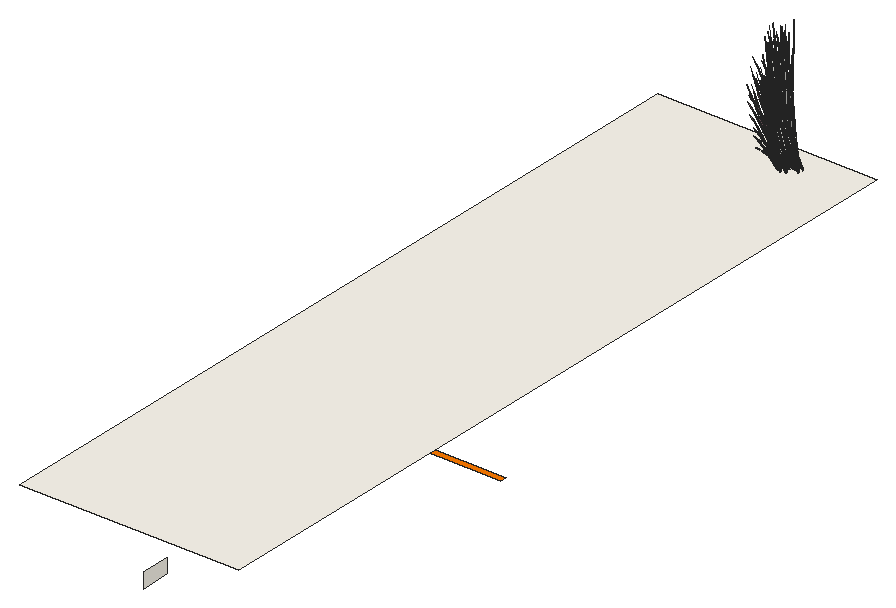
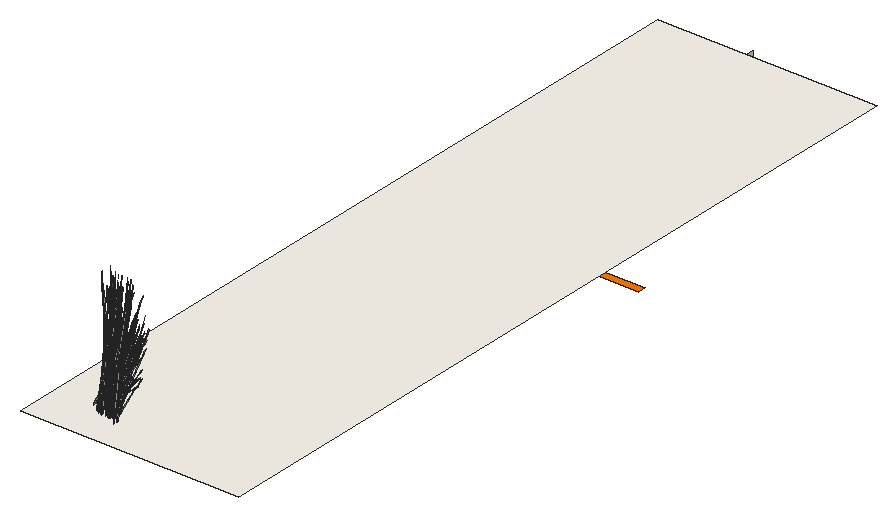
# SketchUp Ruby script. Lengths in inches.
U = 1.inch
M = Sketchup.active_model
def pt(a) = Geom::Point3d.new(a.map { |v| v * U })
def face(e, loops, mat)
  f = e.add_face(loops[0].map { |a| pt(a) })
  loops[1..].each { |l| e.add_face(l.map { |a| pt(a) }).erase! }
  f.material = f.back_material = mat if mat
  f
end
# faces: each face lists its corners as indices into pts; further lists are holes
def faces(e, pts, list, mat = nil) = list.each { |f| face(e, (f[0].is_a?(Array) ? f : [f]).map { |l| l.map { |i| pts[i] } }, mat) }
# xy, xz, yz: faces in a plane at the given z, y or x. An outline is a flat list of corners, or four numbers for a rectangle; further outlines are holes
def ring(l) = l.size == 4 ? [[l[0], l[1]], [l[2], l[1]], [l[2], l[3]], [l[0], l[3]]] : l.each_slice(2).to_a
def flat(e, list, mat, &to3) = list.each { |f| face(e, (f[0].is_a?(Array) ? f : [f]).map { |l| ring(l).map { |u, v| to3.(u, v) } }, mat) }
def xy(e, z, list, mat = nil) = flat(e, list, mat) { |x, y| [x, y, z] }
def xz(e, y, list, mat = nil) = flat(e, list, mat) { |x, z| [x, y, z] }
def yz(e, x, list, mat = nil) = flat(e, list, mat) { |y, z| [x, y, z] }
def lines(e, pts, list) = list.each { |a, b| e.add_line(pt(pts[a]), pt(pts[b])) }
# prism: a flat outline (further loops are holes) pulled along v
def prism(e, loops, v, mat = nil)
  f = face(e, loops, mat); d = Geom::Vector3d.new(v.map { |x| x * U })
  f.pushpull(f.normal.samedirection?(d) ? d.length : -d.length)
end
def box(e, o, s, mat = nil) = prism(e, [[o, [o[0] + s[0], o[1], o[2]], [o[0] + s[0], o[1] + s[1], o[2]], [o[0], o[1] + s[1], o[2]]]], [0, 0, s[2]], mat)
def at(x, y, z, deg = 0) = Geom::Transformation.translation(pt([x, y, z])) * Geom::Transformation.rotation(ORIGIN, Z_AXIS, deg.degrees)
def axes(o, x, y, z) = Geom::Transformation.new([*x, 0, *y, 0, *z, 0, *pt(o).to_a, 1])
def part(name) = M.definitions.add(name)
# library, detail: a bought-in or finely detailed component or shape, given as its bounding box
def library(name, o, s) = part(name).tap { |d| box(d.entities, o, s) }
def detail(e, o, s) = box(e.add_group.entities, o, s)
def put(e, d, t, mat = nil) = e.add_instance(d, t).tap { |i| i.material = mat if mat }
def group(e, t, mat = nil) = e.add_group.tap { |g| g.transformation = t; g.material = mat if mat }.entities
root = M.entities
M.materials.add("C01_Vanilla_Cream").color = [255, 251, 241]
M.materials.add("C05_Golden_Blaze").color = [255, 123, 0]
M.materials.add("LightPink_Translucent").color = [144, 107, 117]
M.materials["LightPink_Translucent"].alpha = 0.75
c1 = part("blade")
p = [[2.15,0.21,22],[0,0.17,0],[0.09,0.45,0],[2.18,0.31,22],[2.29,0.31,22],[0.38,0.45,0],
  [2.48,0.24,33],[2.49,0.24,33],[2.48,0.22,33]]
faces(c1.entities,p,[[0,1,2,3],[4,5,2,3],[6,3,4,7],[8,0,3,6]])
c2 = part("seeds")
p = [[0.3,-0.1,1.38],[-0.01,-0.03,1.59],[-0.01,-0.03,0.03],[0.14,-0.07,-0.07],[0.29,-0.03,3],[0.15,0.01,3.11]]
faces(c2.entities,p,[[0,1,2,3],[1,0,4,5]],"LightPink_Translucent")
c3 = part("blade with seeds")
put(c3.entities,c1,at(0,0,0))
put(c3.entities,c2,axes([2.4,0.25,30.99],[1.5799,-0.05474,1.17369],[-0.12525,1.92788,0.29478],[-0.07173,-0.02425,1.56792]))
xy(root,375,[[603,144,706,146.7]],"C05_Golden_Blaze")
xy(root,390,[[603,24,693.41,354]],"C01_Vanilla_Cream")
yz(root,663.55,[[12,378,24,384]],"C01_Vanilla_Cream")
put(root,c3,axes([666.375,337.75,393.22],[0.14872,0.18332,1.42242],[-0.6872,0.15433,0.11501],[-0.15531,-0.28779,0.60807]))
put(root,c3,axes([670.125,337.75,393.22],[0.14872,0.18332,1.42242],[-0.6872,0.15433,0.11501],[-0.15531,-0.28779,0.60807]))
put(root,c3,axes([667.51,336.54,393.91],[-0.09951,-0.08005,1.45204],[-0.66407,0.05075,-0.22964],[-0.10598,-0.19148,0.11645]))
put(root,c3,axes([668.21,337.89,394.13],[-0.31051,-0.46426,-0.58968],[0.63919,-0.25873,0.07116],[-0.07261,-0.22432,0.83415]))
put(root,c3,axes([666.1875,337.27,392.15],[-0.0394,0.18678,1.18691],[-0.57594,0.15636,-0.25526],[-0.13463,-0.24142,0.50747]))
put(root,c3,axes([669.9375,337.27,392.15],[-0.0394,0.18678,1.18691],[-0.57594,0.15636,-0.25526],[-0.13463,-0.24142,0.50747]))
put(root,c3,axes([667.67,336.86,391.24],[-0.10912,0.02057,1.46364],[-0.60346,-0.23156,-0.2236],[0.01013,-0.19315,0.24931]))
put(root,c3,axes([668.27,337.5,393.76],[0.19614,-0.43908,-0.29394],[0.57222,0.12807,0.37948],[-0.05247,-0.17678,0.72609]))
put(root,c3,axes([667.97,337.8,393.89],[-0.63954,-0.14313,-0.42412],[0.21921,-0.49074,-0.32852],[-0.05864,-0.19758,0.81151]))
put(root,c3,axes([666.83,336.28,393.91],[-0.01214,0.06844,1.47228],[-0.59861,0.24837,-0.13912],[-0.17615,-0.12696,0.26054]))
put(root,c3,axes([670.58,336.28,393.91],[-0.01214,0.06844,1.47228],[-0.59861,0.24837,-0.13912],[-0.17615,-0.12696,0.26054]))
put(root,c3,axes([666.7,337.49,394.23],[0.72473,-0.14676,0.44623],[0.12578,0.57568,0.36794],[-0.17045,-0.16967,0.92337]))
put(root,c3,axes([670.45,337.49,394.23],[0.72473,-0.14676,0.44623],[0.12578,0.57568,0.36794],[-0.17045,-0.16967,0.92337]))
put(root,c3,axes([668.34,337.6,393.93],[0.64106,0.14927,0.39842],[-0.21921,0.49074,0.32852],[-0.03852,-0.19299,0.82444]))
put(root,c3,axes([668.52,337.77,394.18],[-0.63664,0.26583,-0.10093],[-0.31286,-0.47181,-0.56021],[-0.084,-0.19882,0.85122]))
put(root,c3,axes([665.99,336.97,392.3],[0.33937,0.19872,0.95334],[-0.49424,0.11946,0.70045],[-0.10575,-0.15273,0.20998]))
put(root,c3,axes([669.74,336.97,392.3],[0.33937,0.19872,0.95334],[-0.49424,0.11946,0.70045],[-0.10575,-0.15273,0.20998]))
put(root,c3,axes([668.51,337.5625,393.93],[0.47939,-0.19405,0.05337],[0.23464,0.35385,0.42015],[-0.0463,-0.15598,0.64067]))
put(root,c3,axes([666.81,338.02,394.13],[-0.55475,-0.27598,-0.58968],[0.39425,-0.48361,0.07116],[-0.20099,-0.16478,0.83415]))
put(root,c3,axes([670.56,338.02,394.13],[-0.55475,-0.27598,-0.58968],[0.39425,-0.48361,0.07116],[-0.20099,-0.16478,0.83415]))
put(root,c3,axes([666.62,337.66,393.76],[-0.10048,-0.4599,-0.29394],[0.5744,-0.12144,0.37948],[-0.15428,-0.13179,0.72609]))
put(root,c3,axes([670.37,337.66,393.76],[-0.10048,-0.4599,-0.29394],[0.5744,-0.12144,0.37948],[-0.15428,-0.13179,0.72609]))
put(root,c3,axes([666.87,337.62,393.93],[0.29569,-0.36271,0.05337],[0.42107,0.21117,0.42015],[-0.13613,-0.11629,0.64067]))
put(root,c3,axes([670.61,337.62,393.93],[0.29569,-0.36271,0.05337],[0.42107,0.21117,0.42015],[-0.13613,-0.11629,0.64067]))
put(root,c3,axes([665.72,337.57,391.24],[-0.06302,0.07522,1.46364],[-0.63686,0.16217,-0.2236],[-0.15385,-0.14752,0.24931]))
put(root,c3,axes([669.47,337.57,391.24],[-0.06302,0.07522,1.46364],[-0.63686,0.16217,-0.2236],[-0.15385,-0.14752,0.24931]))
put(root,c3,axes([666.77,339.64,391.74],[-0.26718,-0.5855,-0.57963],[0.76964,-0.21087,-0.15213],[-0.02953,-0.19827,1.27944]))
put(root,c3,axes([669.13,338.33,393.22],[0.24166,0.09837,1.42242],[-0.50011,0.41269,0.11501],[-0.3117,-0.18617,0.60807]))
put(root,c3,axes([673.3125,338.33,393.22],[0.24166,0.09837,1.42242],[-0.50011,0.41269,0.11501],[-0.3117,-0.18617,0.60807]))
put(root,c3,axes([668.33,337.96,394.19],[-0.19614,0.43908,0.29394],[-0.57222,-0.12807,-0.37948],[-0.05247,-0.17678,0.72609]))
put(root,c3,axes([666.55,338.04,393.89],[-0.64198,0.13573,-0.42412],[-0.1123,-0.514,-0.32852],[-0.17243,-0.1473,0.81151]))
put(root,c3,axes([670.3,338.04,393.89],[-0.64198,0.13573,-0.42412],[-0.1123,-0.514,-0.32852],[-0.17243,-0.1473,0.81151]))
put(root,c3,axes([667,337.58,394.51],[-0.4342,0.54737,-0.11304],[-0.6288,-0.31535,-0.62743],[-0.21858,-0.15465,0.95337]))
put(root,c3,axes([670.75,337.58,394.51],[-0.4342,0.54737,-0.11304],[-0.6288,-0.31535,-0.62743],[-0.21858,-0.15465,0.95337]))
put(root,c3,axes([667.56,337.26,391.77],[-0.44958,0.32756,-0.03231],[-0.41194,-0.35875,-0.14649],[-0.029,-0.10165,0.48318]))
put(root,c3,axes([669.08,337.42,393.91],[-0.13998,-0.00403,1.45204],[-0.44565,0.40302,-0.22964],[-0.23779,-0.08235,0.11645]))
put(root,c3,axes([673.26,337.42,393.91],[-0.13998,-0.00403,1.45204],[-0.44565,0.40302,-0.22964],[-0.23779,-0.08235,0.11645]))
put(root,c3,axes([668.14,341.15,392.76],[0.56221,0.23024,1.25546],[-0.55078,0.49601,0.49647],[-0.2467,-0.29398,1.05249]))
put(root,c3,axes([671.89,341.15,392.76],[0.56221,0.23024,1.25546],[-0.55078,0.49601,0.49647],[-0.2467,-0.29398,1.05249]))
put(root,c3,axes([666.96,338.03,394.19],[0.10048,0.4599,0.29394],[-0.5744,0.12144,-0.37948],[-0.15428,-0.13179,0.72609]))
put(root,c3,axes([670.71,338.03,394.19],[0.10048,0.4599,0.29394],[-0.5744,0.12144,-0.37948],[-0.15428,-0.13179,0.72609]))
put(root,c3,axes([665.2,339.55,391.67],[0,-0.57097,-0.4121],[0.72788,0,0],[0,-0.13004,1.30728]))
put(root,c3,axes([668.98,338.33,394.23],[0.53728,-0.42137,0.44623],[0.46337,0.44748,0.36794],[-0.25207,-0.07773,0.92337]))
put(root,c3,axes([669.23,338.33,393.93],[0.03276,-0.43418,0.05337],[0.49468,0.0119,0.42015],[-0.18949,-0.04543,0.64067]))
put(root,c3,axes([667.18,339.79,391.83],[0.31565,-0.51449,-0.37133],[0.65588,0.24761,0.17871],[0,-0.1186,1.19224]))
put(root,c3,axes([669.04,338.47,393.76],[-0.37017,-0.35748,-0.29394],[0.42268,-0.3384,0.37948],[-0.21476,-0.05149,0.72609]))
put(root,c3,axes([673.22,338.47,393.76],[-0.37017,-0.35748,-0.29394],[0.42268,-0.3384,0.37948],[-0.21476,-0.05149,0.72609]))
put(root,c3,axes([665.51,339.57,391.68],[0.45414,-0.35624,-0.25712],[0.45414,0.35624,0.25712],[0,-0.11474,1.15348]))
put(root,c3,axes([665.33,337.86,391.77],[-0.18768,0.46622,-0.03231],[-0.57763,-0.14342,-0.14649],[-0.0877,-0.07626,0.48318]))
put(root,c3,axes([669.07,337.86,391.77],[-0.18768,0.46622,-0.03231],[-0.57763,-0.14342,-0.14649],[-0.0877,-0.07626,0.48318]))
put(root,c3,axes([667.1,340.21,392.21],[-0.73268,-0.27244,-0.24149],[0.35279,-0.57501,-0.41502],[-0.02303,-0.14118,1.32557]))
put(root,c3,axes([665.02,339.99,391.97],[-0.81352,0,0],[0,-0.63814,-0.42834],[0,-0.14534,1.3588]))
put(root,c3,axes([668.76,339.99,391.97],[-0.81352,0,0],[0,-0.63814,-0.42834],[0,-0.14534,1.3588]))
put(root,c3,axes([668.9,338.85,392.15],[0.12702,0.15896,1.18691],[-0.2927,0.4321,-0.25526],[-0.30054,-0.10328,0.50747]))
put(root,c3,axes([673.08,338.85,392.15],[0.12702,0.15896,1.18691],[-0.2927,0.4321,-0.25526],[-0.30054,-0.10328,0.50747]))
put(root,c3,axes([669.43,338.71,394.13],[-0.65035,-0.01375,-0.58968],[0.04368,-0.5789,0.07116],[-0.27552,-0.06109,0.83415]))
put(root,c3,axes([673.61,338.71,394.13],[-0.65035,-0.01375,-0.58968],[0.04368,-0.5789,0.07116],[-0.27552,-0.06109,0.83415]))
put(root,c3,axes([665.65,339.82,391.93],[-0.60515,0.48003,0.25528],[-0.60552,-0.47498,-0.30288],[-0.02113,-0.13632,1.36855]))
put(root,c3,axes([669.39,339.82,391.93],[-0.60515,0.48003,0.25528],[-0.60552,-0.47498,-0.30288],[-0.02113,-0.13632,1.36855]))
put(root,c3,axes([668.54,337.76,393.91],[0.04823,0.05698,1.47228],[-0.23252,0.51221,-0.13912],[-0.23548,0.00371,0.26054]))
put(root,c3,axes([672.73,337.76,393.91],[0.04823,0.05698,1.47228],[-0.23252,0.51221,-0.13912],[-0.23548,0.00371,0.26054]))
put(root,c3,axes([667.57,340.04,392.02],[0.73304,0.27674,0.19974],[-0.35279,0.57501,0.41502],[0,-0.13255,1.3325]))
put(root,c3,axes([667.28,340.82,392.02],[0.17244,-0.67657,-0.19446],[0.81759,0.11793,0.42555],[-0.14286,-0.09343,1.29846]))
put(root,c3,axes([671.03,340.82,392.02],[0.17244,-0.67657,-0.19446],[0.81759,0.11793,0.42555],[-0.14286,-0.09343,1.29846]))
put(root,c3,axes([669.21,338.82,393.89],[-0.47241,0.37822,-0.42412],[-0.41372,-0.39954,-0.32852],[-0.24002,-0.05755,0.81151]))
put(root,c3,axes([673.39,338.82,393.89],[-0.47241,0.37822,-0.42412],[-0.41372,-0.39954,-0.32852],[-0.24002,-0.05755,0.81151]))
put(root,c3,axes([665.8125,338.65,394.19],[0.37017,0.35748,0.29394],[-0.42268,0.3384,-0.37948],[-0.21476,-0.05149,0.72609]))
put(root,c3,axes([669.5625,338.65,394.19],[0.37017,0.35748,0.29394],[-0.42268,0.3384,-0.37948],[-0.21476,-0.05149,0.72609]))
put(root,c3,axes([668.15,339.32,392.3],[0.41536,-0.04086,0.95334],[-0.26347,0.35999,0.70045],[-0.20525,-0.054,0.20998]))
put(root,c3,axes([667.33,339.66,392.26],[-0.70648,0.03525,0.37133],[-0.06389,-0.58508,-0.17871],[0.12647,-0.0593,1.19224]))
put(root,c3,axes([669.46,338.43,394.18],[-0.03484,0.58066,-0.10093],[-0.65957,-0.01587,-0.56021],[-0.25402,-0.04034,0.85122]))
put(root,c3,axes([673.64,338.43,394.18],[-0.03484,0.58066,-0.10093],[-0.65957,-0.01587,-0.56021],[-0.25402,-0.04034,0.85122]))
put(root,c3,axes([665.51,340.08,392.06],[0,0.57097,0.4121],[-0.72788,0,0],[0,-0.13004,1.30728]))
put(root,c3,axes([672.8,339.23,393.22],[0.26985,-0.01293,1.42242],[-0.17902,0.56047,0.11501],[-0.38456,-0.03467,0.60807]))
put(root,c3,axes([667.23,340.54,391.83],[-0.39083,-0.47924,-0.37133],[0.59199,-0.33747,0.17871],[-0.12647,-0.0593,1.19224]))
put(root,c3,axes([670.98,340.54,391.83],[-0.39083,-0.47924,-0.37133],[0.59199,-0.33747,0.17871],[-0.12647,-0.0593,1.19224]))
put(root,c3,axes([667.31,339.87,391.96],[0.28286,0.63846,0.37976],[-0.80821,0.22202,0.14902],[0.00988,-0.11732,1.31851]))
put(root,c3,axes([662.04,343.22,392.15],[-0.18493,0.11557,1.18691],[-0.55384,-0.20228,-0.25526],[0.10266,-0.25157,0.50747]))
put(root,c3,axes([667.17,340.37,392.26],[-0.31565,0.51449,0.37133],[-0.65588,-0.24761,-0.17871],[0,-0.1186,1.19224]))
put(root,c3,axes([668.33,339.92,391.83],[0,-0.66065,0],[0.81352,0,0],[0,0,1.48949]))
put(root,c3,axes([670.625,340.73,391.71],[-0.67676,-0.09361,-0.51753],[0.14281,-0.57742,-0.13583],[-0.20196,-0.06997,1.14236]))
put(root,c3,axes([662.49,344.08,394.13],[0.01693,-0.52814,-0.58968],[0.71285,0.03547,0.07116],[0.07523,-0.22375,0.83415]))
put(root,c3,axes([668.53,340.43,391.91],[-0.60515,-0.49144,-0.05089],[0.60552,-0.49174,0],[-0.02113,-0.01716,1.45724]))
put(root,c3,axes([667,338.65,392.05],[-0.18794,0.56744,0.14643],[-0.68774,-0.16058,0.29122],[0.1188,-0.00276,1.33138]))
put(root,c3,axes([663.48,343.25,393.91],[-0.00628,-0.11364,1.45204],[-0.53042,-0.32843,-0.22964],[0.08201,-0.19909,0.11645]))
put(root,c3,axes([661.68,343.81,393.22],[-0.12114,0.19625,1.42242],[-0.50818,-0.40613,0.11501],[0.22925,-0.25313,0.60807]))
put(root,c3,axes([663.34,342.84,393.91],[-0.06607,0.04361,1.47228],[-0.64734,-0.14714,-0.13912],[-0.02343,-0.19032,0.26054]))
put(root,c3,axes([668.51,339.65,393.93],[0.18381,-0.5206,0.39842],[0.60429,0.17802,0.32852],[-0.23764,0.03129,0.82444]))
put(root,c3,axes([672.69,339.65,393.93],[0.18381,-0.5206,0.39842],[0.60429,0.17802,0.32852],[-0.23764,0.03129,0.82444]))
put(root,c3,axes([668.46,339.51,393.93],[-0.23895,-0.38931,0.05337],[0.43573,-0.19055,0.42015],[-0.19208,0.0376,0.64067]))
put(root,c3,axes([672.64,339.51,393.93],[-0.23895,-0.38931,0.05337],[0.43573,-0.19055,0.42015],[-0.19208,0.0376,0.64067]))
put(root,c3,axes([667.38,340.49,391.96],[0.82229,0.1203,0.37976],[-0.16734,0.67942,0.14902],[-0.12017,-0.06561,1.31851]))
put(root,c3,axes([668.45,339.91,391.24],[0.0165,0.08998,1.46364],[-0.33262,0.46992,-0.2236],[-0.23626,-0.02369,0.24931]))
put(root,c3,axes([672.63,339.91,391.24],[0.0165,0.08998,1.46364],[-0.33262,0.46992,-0.2236],[-0.23626,-0.02369,0.24931]))
put(root,c3,axes([662.34,343.9,393.89],[-0.46573,-0.38364,-0.42412],[0.49199,-0.33598,-0.32852],[0.07086,-0.19492,0.81151]))
put(root,c3,axes([666.16,341.61,391.68],[-0.15283,-0.49751,-0.25712],[0.60696,-0.14127,0.25712],[-0.12236,-0.05737,1.15348]))
put(root,c3,axes([669.91,341.61,391.68],[-0.15283,-0.49751,-0.25712],[0.60696,-0.14127,0.25712],[-0.12236,-0.05737,1.15348]))
put(root,c3,axes([666.9375,341.58,392.05],[0.6991,-0.15154,0.14643],[0.17263,0.56398,0.29122],[-0.06235,-0.08217,1.33138]))
put(root,c3,axes([665.99,341.82,391.67],[-0.60889,-0.28548,-0.4121],[0.36394,-0.51192,0],[-0.13868,-0.06502,1.30728]))
put(root,c3,axes([669.74,341.82,391.67],[-0.60889,-0.28548,-0.4121],[0.36394,-0.51192,0],[-0.13868,-0.06502,1.30728]))
put(root,c3,axes([668.38,339.71,393.76],[-0.54068,-0.15928,-0.29394],[0.1577,-0.46469,0.37948],[-0.21769,0.04261,0.72609]))
put(root,c3,axes([672.5625,339.71,393.76],[-0.54068,-0.15928,-0.29394],[0.1577,-0.46469,0.37948],[-0.21769,0.04261,0.72609]))
put(root,c3,axes([662.83,344.1,394.18],[-0.71502,-0.02829,-0.10093],[0.01954,-0.53563,-0.56021],[0.04967,-0.20629,0.85122]))
put(root,c3,axes([662.78,343.76,393.76],[0.4402,-0.30062,-0.29394],[0.41671,0.34326,0.37948],[0.0634,-0.1744,0.72609]))
put(root,c3,axes([667.64,340.8125,392.21],[-0.65687,0.37907,-0.24149],[-0.43681,-0.53562,-0.41502],[-0.16207,-0.0544,1.32557]))
put(root,c3,axes([671.39,340.8125,392.21],[-0.65687,0.37907,-0.24149],[-0.43681,-0.53562,-0.41502],[-0.16207,-0.0544,1.32557]))
put(root,c3,axes([667.99,341.45,391.83],[-0.21227,-0.49226,0],[0.60616,-0.17239,0],[0,0,1.28128]))
put(root,c3,axes([667.58,340.98,392.17],[-0.12551,0.50956,0.12018],[-0.6132,-0.08845,-0.34318],[-0.1116,-0.05232,1.05198]))
put(root,c3,axes([671.33,340.98,392.17],[-0.12551,0.50956,0.12018],[-0.6132,-0.08845,-0.34318],[-0.1116,-0.05232,1.05198]))
put(root,c3,axes([668.95,339.66,394.19],[0.54068,0.15928,0.29394],[-0.1577,0.46469,-0.37948],[-0.21769,0.04261,0.72609]))
put(root,c3,axes([669.02,341.61,392.05],[0.18794,-0.56744,0.14643],[0.68774,0.16058,0.29122],[-0.1188,0.00276,1.33138]))
put(root,c3,axes([663.33,343.58,391.24],[-0.09738,-0.04498,1.46364],[-0.25012,-0.50252,-0.2236],[0.16873,-0.13637,0.24931]))
put(root,c3,axes([670.03,339.63,392.77],[0.18493,-0.0826,1.46963],[0.06377,0.5767,0.11501],[-0.40056,0.07652,0.52526]))
put(root,c3,axes([674.21,339.63,392.77],[0.18493,-0.0826,1.46963],[0.06377,0.5767,0.11501],[-0.40056,0.07652,0.52526]))
put(root,c3,axes([670.09,340.16,392.05],[-0.51116,-0.4159,0.14643],[0.51512,-0.4034,0.29122],[-0.05645,0.08494,1.33138]))
put(root,c3,axes([667.84,341.67,391.82],[-0.65588,-0.25634,0],[0.31565,-0.53263,0],[0,0,1.35047]))
put(root,c3,axes([668.38,340.99,392.05],[-0.63528,-0.45956,-0.20909],[0.53456,-0.51604,0.45758],[-0.17107,0.05376,1.39619]))
put(root,c3,axes([672.13,340.99,392.05],[-0.63528,-0.45956,-0.20909],[0.53456,-0.51604,0.45758],[-0.17107,0.05376,1.39619]))
put(root,c3,axes([662.78,343.88,393.93],[0.46327,0.38957,0.39842],[-0.49199,0.33598,0.32852],[0.08546,-0.18277,0.82444]))
put(root,c3,axes([666.71,341.87,392.06],[0.60889,0.28548,0.4121],[-0.36394,0.51192,0],[-0.13868,-0.06502,1.30728]))
put(root,c3,axes([670.46,341.87,392.06],[0.60889,0.28548,0.4121],[-0.36394,0.51192,0],[-0.13868,-0.06502,1.30728]))
put(root,c3,axes([662.95,343.91,393.93],[0.53464,0.0266,0.05337],[-0.01466,0.40172,0.42015],[0.05594,-0.15388,0.64067]))
put(root,c3,axes([662.55,344.1875,394.19],[-0.4402,0.30062,0.29394],[-0.41671,-0.34326,-0.37948],[0.0634,-0.1744,0.72609]))
put(root,c3,axes([663.33,345,394.13],[0.33983,-0.45051,-0.58968],[0.59551,0.32017,0.07116],[0.20291,-0.16322,0.83415]))
put(root,c3,axes([663.31,344.79,393.89],[-0.16713,-0.52135,-0.42412],[0.63294,-0.0912,-0.32852],[0.18138,-0.14003,0.81151]))
put(root,c3,axes([668.04,340.02,393.91],[-0.10624,0.07413,1.45204],[0.00904,0.54162,-0.22964],[-0.24352,0.07044,0.11645]))
put(root,c3,axes([672.22,340.02,393.91],[-0.10624,0.07413,1.45204],[0.00904,0.54162,-0.22964],[-0.24352,0.07044,0.11645]))
put(root,c3,axes([668.73,340.19,391.9],[0,0.66033,-0.04679],[-0.81352,0,0],[0,0.02075,1.48875]))
put(root,c3,axes([668.75,339.94,393.89],[-0.17625,0.51936,-0.42412],[-0.60429,-0.17802,-0.32852],[-0.2433,0.04762,0.81151]))
put(root,c3,axes([672.94,339.94,393.89],[-0.17625,0.51936,-0.42412],[-0.60429,-0.17802,-0.32852],[-0.2433,0.04762,0.81151]))
put(root,c3,axes([668.72,339.5,394.18],[0.32734,0.51701,-0.10093],[-0.58097,0.25407,-0.56021],[-0.24483,0.06821,0.85122]))
put(root,c3,axes([672.91,339.5,394.18],[0.32734,0.51701,-0.10093],[-0.58097,0.25407,-0.56021],[-0.24483,0.06821,0.85122]))
put(root,c3,axes([666.36,342.17,391.97],[-0.40676,0.57214,0],[-0.68052,-0.31907,-0.42834],[-0.15499,-0.07267,1.3588]))
